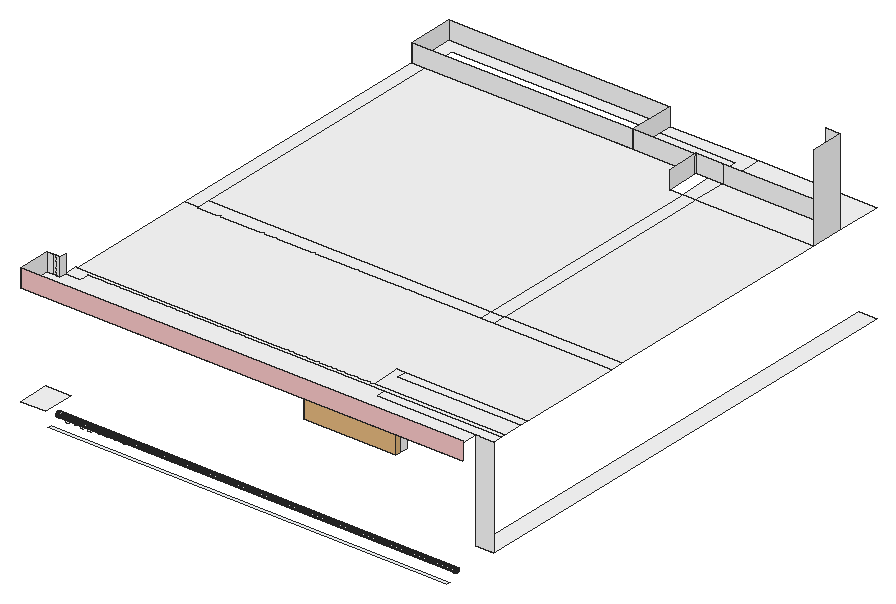
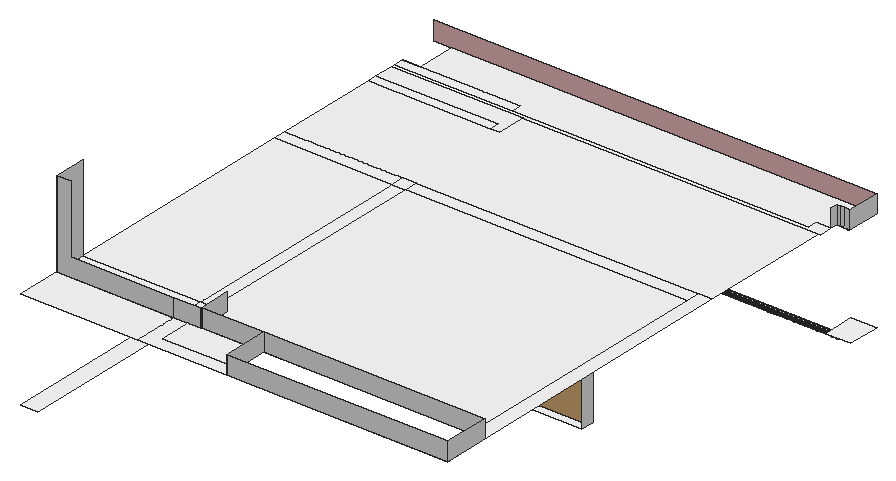
# SketchUp Ruby script. Lengths in inches.
U = 1.inch
M = Sketchup.active_model
def pt(a) = Geom::Point3d.new(a.map { |v| v * U })
def face(e, loops, mat)
  f = e.add_face(loops[0].map { |a| pt(a) })
  loops[1..].each { |l| e.add_face(l.map { |a| pt(a) }).erase! }
  f.material = f.back_material = mat if mat
  f
end
# faces: each face lists its corners as indices into pts; further lists are holes
def faces(e, pts, list, mat = nil) = list.each { |f| face(e, (f[0].is_a?(Array) ? f : [f]).map { |l| l.map { |i| pts[i] } }, mat) }
# xy, xz, yz: faces in a plane at the given z, y or x. An outline is a flat list of corners, or four numbers for a rectangle; further outlines are holes
def ring(l) = l.size == 4 ? [[l[0], l[1]], [l[2], l[1]], [l[2], l[3]], [l[0], l[3]]] : l.each_slice(2).to_a
def flat(e, list, mat, &to3) = list.each { |f| face(e, (f[0].is_a?(Array) ? f : [f]).map { |l| ring(l).map { |u, v| to3.(u, v) } }, mat) }
def xy(e, z, list, mat = nil) = flat(e, list, mat) { |x, y| [x, y, z] }
def xz(e, y, list, mat = nil) = flat(e, list, mat) { |x, z| [x, y, z] }
def yz(e, x, list, mat = nil) = flat(e, list, mat) { |y, z| [x, y, z] }
def lines(e, pts, list) = list.each { |a, b| e.add_line(pt(pts[a]), pt(pts[b])) }
# prism: a flat outline (further loops are holes) pulled along v
def prism(e, loops, v, mat = nil)
  f = face(e, loops, mat); d = Geom::Vector3d.new(v.map { |x| x * U })
  f.pushpull(f.normal.samedirection?(d) ? d.length : -d.length)
end
def box(e, o, s, mat = nil) = prism(e, [[o, [o[0] + s[0], o[1], o[2]], [o[0] + s[0], o[1] + s[1], o[2]], [o[0], o[1] + s[1], o[2]]]], [0, 0, s[2]], mat)
def at(x, y, z, deg = 0) = Geom::Transformation.translation(pt([x, y, z])) * Geom::Transformation.rotation(ORIGIN, Z_AXIS, deg.degrees)
def axes(o, x, y, z) = Geom::Transformation.new([*x, 0, *y, 0, *z, 0, *pt(o).to_a, 1])
def part(name) = M.definitions.add(name)
# library, detail: a bought-in or finely detailed component or shape, given as its bounding box
def library(name, o, s) = part(name).tap { |d| box(d.entities, o, s) }
def detail(e, o, s) = box(e.add_group.entities, o, s)
def put(e, d, t, mat = nil) = e.add_instance(d, t).tap { |i| i.material = mat if mat }
def group(e, t, mat = nil) = e.add_group.tap { |g| g.transformation = t; g.material = mat if mat }.entities
root = M.entities
M.materials.add("A01_Blush_Petal").color = [255, 204, 204]
M.materials.add("Glass_Basic_01").color = [161, 173, 186]
M.materials["Glass_Basic_01"].alpha = 0.25
M.materials.add("M00_Soft_Cloud").color = [255, 255, 255]
c1 = library("Group\#30",[0,0,0],[77.46,3.16,80.98])
xy(root,282.07,[[278.74,261.09,340.22,270.09]],"M00_Soft_Cloud")
xy(root,304.79,[[205.78,138.3,472.6,141.64]],"Glass_Basic_01")
xy(root,308.51,[[219.09,145.24,219.51,145.29,219.89,145.45,220.22,145.7,220.48,146.03,220.64,146.42,220.69,146.83,220.64,147.25,220.48,147.63,220.22,147.96,219.89,148.22,219.51,148.38,219.09,148.43,218.68,148.38,218.29,148.22,217.96,147.96,217.71,147.63,217.55,147.25,217.5,146.83,217.55,146.42,217.71,146.03,217.96,145.7,218.29,145.45,218.68,145.29]],"M00_Soft_Cloud")
xy(root,308.55,[[251.01,145.24,251.42,145.29,251.8,145.45,252.14,145.7,252.39,146.03,252.55,146.42,252.6,146.83,252.55,147.25,252.39,147.63,252.14,147.96,251.8,148.22,251.42,148.38,251.01,148.43,250.59,148.38,250.21,148.22,249.875,147.96,249.62,147.63,249.46,147.25,249.41,146.83,249.46,146.42,249.62,146.03,249.875,145.7,250.21,145.45,250.59,145.29]],"M00_Soft_Cloud")
xy(root,308.6875,[[239.53,145.24,239.95,145.29,240.33,145.45,240.66,145.7,240.92,146.03,241.08,146.42,241.13,146.83,241.08,147.25,240.92,147.63,240.66,147.96,240.33,148.22,239.95,148.38,239.53,148.43,239.12,148.38,238.73,148.22,238.4,147.96,238.15,147.63,237.99,147.25,237.9375,146.83,237.99,146.42,238.15,146.03,238.4,145.7,238.73,145.45,239.12,145.29]],"M00_Soft_Cloud")
xy(root,308.83,[[234.29,145.24,234.7,145.29,235.09,145.45,235.3125,145.625,233.26,145.625,233.49,145.45,233.875,145.29],[245.47,145.24,245.88,145.29,246.27,145.45,246.5,145.625,244.44,145.625,244.67,145.45,245.06,145.29],[233.26,145.625,235.3125,145.625,235.42,145.7,235.67,146.03,235.83,146.42,235.89,146.83,235.83,147.25,235.67,147.63,235.42,147.96,235.09,148.22,234.7,148.38,234.6,148.39,233.98,148.39,233.875,148.38,233.49,148.22,233.16,147.96,232.9,147.63,232.74,147.25,232.6875,146.83,232.74,146.42,232.9,146.03,233.16,145.7],[244.44,145.625,246.5,145.625,246.6,145.7,246.85,146.03,247.01,146.42,247.07,146.83,247.01,147.25,246.85,147.63,246.6,147.96,246.27,148.22,245.88,148.38,245.78,148.39,245.16,148.39,245.06,148.38,244.67,148.22,244.34,147.96,244.09,147.63,243.93,147.25,243.87,146.83,243.93,146.42,244.09,146.03,244.34,145.7],[233.98,148.39,234.6,148.39,234.29,148.43],
  [245.16,148.39,245.78,148.39,245.47,148.43]],"M00_Soft_Cloud")
xy(root,309.4375,[[274.92,145.24,275.33,145.29,275.72,145.45,276.05,145.7,276.3,146.03,276.46,146.42,276.52,146.83,276.46,147.25,276.3,147.63,276.05,147.96,275.72,148.22,275.33,148.38,274.92,148.43,274.5,148.38,274.12,148.22,273.79,147.96,273.53,147.63,273.375,147.25,273.32,146.83,273.375,146.42,273.53,146.03,273.79,145.7,274.12,145.45,274.5,145.29]],"M00_Soft_Cloud")
xy(root,309.52,[[256.81,145.24,257.22,145.29,257.61,145.45,257.9375,145.7,258.19,146.03,258.35,146.42,258.41,146.83,258.35,147.25,258.19,147.63,257.9375,147.96,257.61,148.22,257.22,148.38,256.81,148.43,256.39,148.38,256.01,148.22,255.68,147.96,255.42,147.63,255.26,147.25,255.21,146.83,255.26,146.42,255.42,146.03,255.68,145.7,256.01,145.45,256.39,145.29],[268.95,145.24,269.36,145.29,269.75,145.45,270.08,145.7,270.33,146.03,270.49,146.42,270.55,146.83,270.49,147.25,270.33,147.63,270.08,147.96,269.75,148.22,269.36,148.38,268.95,148.43,268.54,148.38,268.15,148.22,267.82,147.96,267.57,147.63,267.41,147.25,267.35,146.83,267.41,146.42,267.57,146.03,267.82,145.7,268.15,145.45,268.54,145.29]],"M00_Soft_Cloud")
xy(root,309.59,[[262.56,145.24,262.98,145.29,263.36,145.45,263.69,145.7,263.95,146.03,264.11,146.42,264.16,146.83,264.11,147.25,263.95,147.63,263.69,147.96,263.36,148.22,262.98,148.38,262.56,148.43,262.15,148.38,261.77,148.22,261.43,147.96,261.18,147.63,261.02,147.25,260.97,146.83,261.02,146.42,261.18,146.03,261.43,145.7,261.77,145.45,262.15,145.29]],"M00_Soft_Cloud")
xy(root,309.83,[[280.99,145.24,281.4,145.29,281.79,145.45,282.12,145.7,282.37,146.03,282.53,146.42,282.59,146.83,282.53,147.25,282.37,147.63,282.12,147.96,281.79,148.22,281.4,148.38,280.99,148.43,280.58,148.38,280.19,148.22,279.86,147.96,279.6,147.63,279.45,147.25,279.39,146.83,279.45,146.42,279.6,146.03,279.86,145.7,280.19,145.45,280.58,145.29]],"M00_Soft_Cloud")
xy(root,315.86,[[189,136.44,205.78,157.97]],"M00_Soft_Cloud")
xy(root,317.36,[[472.6,162.91,484.6,482.39]],"M00_Soft_Cloud")
xy(root,348,[[278.74,261.09,340.22,270.09]],"M00_Soft_Cloud")
xy(root,384,[[189,136.44,189,158.3,198,158.3,198,162.91,208,162.91,208,169.29,405.98,169.29,405.98,162.91,472.6,162.91,472.6,136.44],[189,158.3,198,158.41],[198,162.91,208,162.91,208,169.29,484.6,169.29,484.6,171.91,198,171.91],[405.98,162.91,484.6,169.29],[199,171.91,396.98,171.91,396.98,191.46,484.6,191.46,484.6,261.09,199,261.09],
  [396.98,171.91,484.6,171.91,484.6,185.07,402.59,185.07,402.59,191.46,396.98,191.46],[402.59,185.07,484.6,191.46],[199,261.09,208,451.29],[208,261.09,396.98,270.09],[396.98,261.09,405.98,270.09],
  [405.98,261.09,484.6,270.09],[208,270.09,396.98,270.09,396.98,429.82,388.44,429.82,388.44,451.29,208,451.29],[396.98,270.09,405.98,429.82],[405.98,270.09,484.6,429.82],[396.98,429.82,405.98,451.98],
  [405.98,429.82,484.6,451.98],[199,451.29,208,451.29,208,473.39,346.72,473.39,346.72,482.39,199,482.39],[346.72,451.29,388.44,451.29,388.44,451.98,396.98,451.98,396.98,473.39,346.72,473.39],[396.98,451.98,405.98,451.98,405.98,482.39,346.72,482.39,346.72,473.39,396.98,473.39],[405.98,451.98,484.6,482.39]],"M00_Soft_Cloud")
xz(root,136.44,[[189,384,484.6,396]],"A01_Blush_Petal")
xz(root,158.3,[[189,384,193,396],[193,384,195,396],[195,384,198,396]],"M00_Soft_Cloud")
xz(root,162.91,[[472.6,317.36,484.6,384]],"M00_Soft_Cloud")
xz(root,451.29,[[199,384,346.72,396],[346.72,384,388.44,396]],"M00_Soft_Cloud")
xz(root,451.98,[[388.44,384,405.98,396],[405.98,384,405.98,396,475.23,396,475.23,441.51,484.6,441.51,484.6,384]],"M00_Soft_Cloud")
xz(root,482.39,[[199,384,346.72,396]],"M00_Soft_Cloud")
yz(root,189,[[136.44,384,158.3,396]],"M00_Soft_Cloud")
yz(root,198,[[158.3,384,162.91,396]],"M00_Soft_Cloud")
yz(root,199,[[451.29,384,482.39,396]],"M00_Soft_Cloud")
yz(root,208,[[147.01,308.03,146.59,308.09,146.21,308.25,145.88,308.5,145.625,308.83,145.46,309.22,145.41,309.63,145.46,310.05,145.625,310.43,145.88,310.76,146.21,311.02,146.59,311.18,147.01,311.23,147.42,311.18,147.81,311.02,148.14,310.76,148.39,310.43,148.55,310.05,148.61,309.63,148.55,309.22,148.39,308.83,148.14,308.5,147.81,308.25,147.42,308.09]],"M00_Soft_Cloud")
yz(root,278.74,[[261.09,282.07,270.09,348]],"M00_Soft_Cloud")
yz(root,340.22,[[261.09,282.07,270.09,348]],"M00_Soft_Cloud")
yz(root,346.72,[[451.29,384,482.39,396]],"M00_Soft_Cloud")
yz(root,388.44,[[429.82,384,451.29,396],[451.29,384,451.98,396]],"M00_Soft_Cloud")
yz(root,484.6,[[429.82,384,451.98,441.51]],"M00_Soft_Cloud")
p = [[208,147.01,308.03],[208,146.59,308.09],[205.78,146.59,308.09],[205.78,147.01,308.03],[472.6,147.01,308.03],[472.6,146.59,308.09],
  [208,147.42,308.09],[205.78,147.42,308.09],[472.6,147.42,308.09],[208,146.21,308.25],[205.78,146.21,308.25],[472.6,146.21,308.25],
  [208,147.81,308.25],[205.78,147.81,308.25],[472.6,147.81,308.25],[208,145.88,308.5],[205.78,145.88,308.5],[472.6,145.88,308.5],
  [208,148.14,308.5],[205.78,148.14,308.5],[472.6,148.14,308.5],[208,145.625,308.83],[205.78,145.625,308.83],[472.6,145.625,308.83],
  [246.5,145.625,308.83],[244.44,145.625,308.83],[235.3125,145.625,308.83],[233.26,145.625,308.83],[230.62,145.625,308.83],[229.02,145.625,308.83],
  [227.42,145.625,308.83],[225.56,145.625,308.83],[223.96,145.625,308.83],[222.36,145.625,308.83],[215.71,145.625,308.83],[214.11,145.625,308.83],
  [212.51,145.625,308.83],[208,148.39,308.83],[205.78,148.39,308.83],[233.98,148.39,308.83],[234.6,148.39,308.83],[245.16,148.39,308.83],
  [245.78,148.39,308.83],[472.6,148.39,308.83],[212.57,145.21,308.82],[215.65,145.21,308.82],[215.49,144.83,308.8125],[215.24,144.49,308.8],
  [214.91,144.24,308.8],[214.52,144.08,308.79],[214.11,144.03,308.79],[213.7,144.08,308.79],[213.3125,144.24,308.8],[212.98,144.49,308.8],
  [212.73,144.83,308.8125],[222.41,145.21,308.82],[222.57,144.83,308.8125],[222.83,144.49,308.8],[223.16,144.24,308.8],[223.54,144.08,308.79],
  [223.96,144.03,308.79],[224.37,144.08,308.79],[224.76,144.24,308.8],[225.09,144.49,308.8],[225.34,144.83,308.8125],[225.5,145.21,308.82],
  [227.48,145.21,308.82],[230.5625,145.21,308.82],[230.4,144.83,308.8125],[230.15,144.49,308.8],[229.82,144.24,308.8],[229.43,144.08,308.79],
  [229.02,144.03,308.79],[228.61,144.08,308.79],[228.22,144.24,308.8],[227.89,144.49,308.8],[227.64,144.83,308.8125],[208,145.46,309.22],
  [205.78,145.46,309.22],[472.6,145.46,309.22],[215.65,146.04,308.84],[215.49,146.42,308.85],[215.24,146.75,308.86],[214.91,147.01,308.87],
  [214.52,147.17,308.875],[214.11,147.22,308.875],[213.7,147.17,308.875],[213.3125,147.01,308.87],[212.98,146.75,308.86],[212.73,146.42,308.85],
  [212.57,146.04,308.84],[225.5,146.04,308.84],[222.41,146.04,308.84],[222.57,146.42,308.85],[222.83,146.75,308.86],[223.16,147.01,308.87],
  [223.54,147.17,308.875],[223.96,147.22,308.875],[224.37,147.17,308.875],[224.76,147.01,308.87],[225.09,146.75,308.86],[225.34,146.42,308.85],
  [230.5625,146.04,308.84],[230.4,146.42,308.85],[230.15,146.75,308.86],[229.82,147.01,308.87],[229.43,147.17,308.875],[229.02,147.22,308.875],
  [228.61,147.17,308.875],[228.22,147.01,308.87],[227.89,146.75,308.86],[227.64,146.42,308.85],[227.48,146.04,308.84],[208,148.55,309.22],
  [205.78,148.55,309.22],[472.6,148.55,309.22],[208,145.41,309.63],[205.78,145.41,309.63],[472.6,145.41,309.63],[208,148.61,309.63],
  [205.78,148.61,309.63],[472.6,148.61,309.63],[208,145.46,310.05],[205.78,145.46,310.05],[472.6,145.46,310.05],[208,148.55,310.05],
  [205.78,148.55,310.05],[472.6,148.55,310.05],[208,145.625,310.43],[205.78,145.625,310.43],[472.6,145.625,310.43],[208,148.39,310.43],
  [205.78,148.39,310.43],[472.6,148.39,310.43],[208,145.88,310.76],[205.78,145.88,310.76],[472.6,145.88,310.76],[208,148.14,310.76],
  [205.78,148.14,310.76],[472.6,148.14,310.76],[208,146.21,311.02],[205.78,146.21,311.02],[472.6,146.21,311.02],[208,147.81,311.02],
  [205.78,147.81,311.02],[472.6,147.81,311.02],[208,146.59,311.18],[205.78,146.59,311.18],[472.6,146.59,311.18],[208,147.42,311.18],
  [205.78,147.42,311.18],[472.6,147.42,311.18],[208,147.01,311.23],[205.78,147.01,311.23],[472.6,147.01,311.23],[208,147.01,309.63],
  [472.6,147.01,309.63],[63.82,154.91,387.8125],[63.09,154.91,387.8125]]
faces(root,p,[[0,1,2,3],[1,0,4,5],[6,0,3,7],[0,6,8,4],[1,9,10,2],[9,1,5,11],[12,6,7,13],[6,12,14,8],
  [9,15,16,10],[15,9,11,17],[18,12,13,19],[12,18,20,14],[15,21,22,16],[21,15,17,23,24,25,26,27,28,29,30,31,32,33,34,35,36],[37,18,19,38],[18,37,39,40,41,42,43,20],
  [44,36,35,34,45,46,47,48,49,50,51,52,53,54],[33,55,56,57,58,59,60,61,62,63,64,65,31,32],[66,30,29,28,67,68,69,70,71,72,73,74,75,76],[21,77,78,22],[77,21,36,35,34,33,32,31,30,29,28,27,26,25,24,23,79],[34,80,81,82,83,84,85,86,87,88,89,90,36,35],[91,31,32,33,92,93,94,95,96,97,98,99,100,101],[28,102,103,104,105,106,107,108,109,110,111,112,30,29],
  [113,37,38,114],[37,113,115,43,42,41,40,39],[77,116,117,78],[116,77,79,118],[119,113,114,120],[113,119,121,115],[116,122,123,117],[122,116,118,124],
  [125,119,120,126],[119,125,127,121],[122,128,129,123],[128,122,124,130],[131,125,126,132],[125,131,133,127],[128,134,135,129],[134,128,130,136],
  [137,131,132,138],[131,137,139,133],[134,140,141,135],[140,134,136,142],[143,137,138,144],[137,143,145,139],[140,146,147,141],[146,140,142,148],
  [149,143,144,150],[143,149,151,145],[146,152,153,147],[152,146,148,154],[152,149,150,153],[149,152,154,151]],"M00_Soft_Cloud")
lines(root,p,[[155,156],[157,158]])
put(root,c1,axes([278.74,261.09,282.07],[0.7979,0,0],[0,1,0],[0,0,0.81417]))
